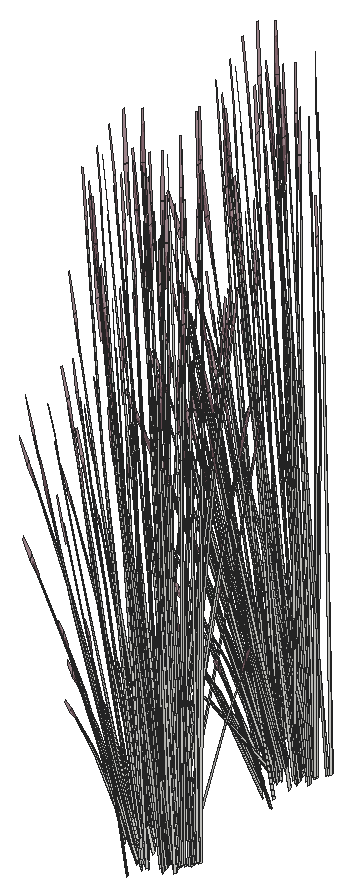
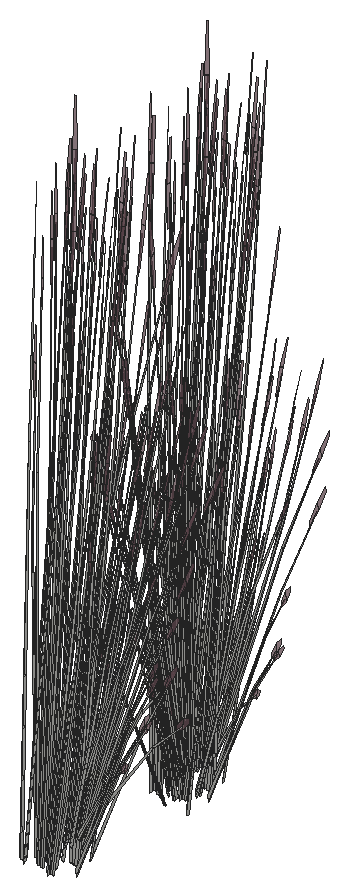
# SketchUp Ruby script. Lengths in inches.
U = 1.inch
M = Sketchup.active_model
def pt(a) = Geom::Point3d.new(a.map { |v| v * U })
def face(e, loops, mat)
  f = e.add_face(loops[0].map { |a| pt(a) })
  loops[1..].each { |l| e.add_face(l.map { |a| pt(a) }).erase! }
  f.material = f.back_material = mat if mat
  f
end
# faces: each face lists its corners as indices into pts; further lists are holes
def faces(e, pts, list, mat = nil) = list.each { |f| face(e, (f[0].is_a?(Array) ? f : [f]).map { |l| l.map { |i| pts[i] } }, mat) }
# xy, xz, yz: faces in a plane at the given z, y or x. An outline is a flat list of corners, or four numbers for a rectangle; further outlines are holes
def ring(l) = l.size == 4 ? [[l[0], l[1]], [l[2], l[1]], [l[2], l[3]], [l[0], l[3]]] : l.each_slice(2).to_a
def flat(e, list, mat, &to3) = list.each { |f| face(e, (f[0].is_a?(Array) ? f : [f]).map { |l| ring(l).map { |u, v| to3.(u, v) } }, mat) }
def xy(e, z, list, mat = nil) = flat(e, list, mat) { |x, y| [x, y, z] }
def xz(e, y, list, mat = nil) = flat(e, list, mat) { |x, z| [x, y, z] }
def yz(e, x, list, mat = nil) = flat(e, list, mat) { |y, z| [x, y, z] }
def lines(e, pts, list) = list.each { |a, b| e.add_line(pt(pts[a]), pt(pts[b])) }
# prism: a flat outline (further loops are holes) pulled along v
def prism(e, loops, v, mat = nil)
  f = face(e, loops, mat); d = Geom::Vector3d.new(v.map { |x| x * U })
  f.pushpull(f.normal.samedirection?(d) ? d.length : -d.length)
end
def box(e, o, s, mat = nil) = prism(e, [[o, [o[0] + s[0], o[1], o[2]], [o[0] + s[0], o[1] + s[1], o[2]], [o[0], o[1] + s[1], o[2]]]], [0, 0, s[2]], mat)
def at(x, y, z, deg = 0) = Geom::Transformation.translation(pt([x, y, z])) * Geom::Transformation.rotation(ORIGIN, Z_AXIS, deg.degrees)
def axes(o, x, y, z) = Geom::Transformation.new([*x, 0, *y, 0, *z, 0, *pt(o).to_a, 1])
def part(name) = M.definitions.add(name)
# library, detail: a bought-in or finely detailed component or shape, given as its bounding box
def library(name, o, s) = part(name).tap { |d| box(d.entities, o, s) }
def detail(e, o, s) = box(e.add_group.entities, o, s)
def put(e, d, t, mat = nil) = e.add_instance(d, t).tap { |i| i.material = mat if mat }
def group(e, t, mat = nil) = e.add_group.tap { |g| g.transformation = t; g.material = mat if mat }.entities
root = M.entities
M.materials.add("LightPink_Translucent").color = [144, 107, 117]
M.materials["LightPink_Translucent"].alpha = 0.75
c1 = part("blade")
p = [[2.15,0.21,22],[0,0.17,0],[0.09,0.45,0],[2.18,0.31,22],[2.29,0.31,22],[0.38,0.45,0],
  [2.48,0.24,33],[2.49,0.24,33],[2.48,0.22,33]]
faces(c1.entities,p,[[0,1,2,3],[4,5,2,3],[6,3,4,7],[8,0,3,6]])
c2 = part("seeds")
p = [[0.3,-0.1,1.38],[-0.01,-0.03,1.59],[-0.01,-0.03,0.03],[0.14,-0.07,-0.07],[0.29,-0.03,3],[0.15,0.01,3.11]]
faces(c2.entities,p,[[0,1,2,3],[1,0,4,5]],"LightPink_Translucent")
c3 = part("blade with seeds")
put(c3.entities,c1,at(0,0,0))
put(c3.entities,c2,axes([2.4,0.25,30.99],[1.5799,-0.05474,1.17369],[-0.12525,1.92788,0.29478],[-0.07173,-0.02425,1.56792]))
put(root,c3,axes([415.25,622.47,157.125],[0.16998,-0.01068,1.44779],[-0.11276,0.46299,0.11706],[-0.24224,-0.02864,0.61892]))
put(root,c3,axes([415.25,635.43,157.55],[0.16998,-0.01068,1.44779],[-0.11276,0.46299,0.11706],[-0.24224,-0.02864,0.61892]))
put(root,c3,axes([415.32,623.29,157.125],[0.14219,-0.09977,1.44779],[0.11971,0.461,0.11706],[-0.22323,0.10419,0.61892]))
put(root,c3,axes([415.32,636.25,157.55],[0.14219,-0.09977,1.44779],[0.11971,0.461,0.11706],[-0.22323,0.10419,0.61892]))
put(root,c3,axes([414.88,624.07,156.04],[0.14242,0.03872,1.20808],[0.09179,0.39548,-0.25981],[-0.19345,0.07403,0.51652]))
put(root,c3,axes([416.14,622.81,156.67],[0.11649,-0.06823,1.49584],[0.04017,0.47639,0.11706],[-0.25231,0.06321,0.53462]))
put(root,c3,axes([416.14,635.77,157.1],[0.11649,-0.06823,1.49584],[0.04017,0.47639,0.11706],[-0.25231,0.06321,0.53462]))
put(root,c3,axes([414.89,623.125,157.83],[-0.06692,0.06124,1.47793],[0.00569,0.44742,-0.23373],[-0.15339,0.05818,0.11853]))
put(root,c3,axes([414.89,636.09,158.26],[-0.06692,0.06124,1.47793],[0.00569,0.44742,-0.23373],[-0.15339,0.05818,0.11853]))
put(root,c3,axes([415.76,622.04,158.06],[-0.40965,-0.01136,-0.60019],[0.02751,-0.47821,0.07243],[-0.17355,-0.05047,0.84903]))
put(root,c3,axes([415.76,635,158.48],[-0.40965,-0.01136,-0.60019],[0.02751,-0.47821,0.07243],[-0.17355,-0.05047,0.84903]))
put(root,c3,axes([415.43,622.16,156.04],[0.08001,0.13132,1.20808],[-0.18437,0.35694,-0.25981],[-0.18931,-0.08532,0.51652]))
put(root,c3,axes([415.43,635.12,156.46],[0.08001,0.13132,1.20808],[-0.18437,0.35694,-0.25981],[-0.18931,-0.08532,0.51652]))
put(root,c3,axes([415.1,622.87,157.68],[-0.34057,-0.13158,-0.29918],[0.09933,-0.38387,0.38624],[-0.13712,0.0352,0.73904]))
put(root,c3,axes([415.1,635.83,158.1],[-0.34057,-0.13158,-0.29918],[0.09933,-0.38387,0.38624],[-0.13712,0.0352,0.73904]))
put(root,c3,axes([415.57,634.69,157.55],[0.15222,0.08126,1.44779],[-0.31502,0.34091,0.11706],[-0.19634,-0.15379,0.61892]))
put(root,c3,axes([414.14,623.58,157.83],[0.0523,0.01265,1.49853],[0.16179,0.41674,-0.1416],[-0.10706,0.10938,0.26519]))
put(root,c3,axes([415.34,623.07,157.81],[-0.11102,0.42903,-0.43168],[-0.38064,-0.14706,-0.33437],[-0.15325,0.03934,0.82598]))
put(root,c3,axes([415.34,636.03,158.23],[-0.11102,0.42903,-0.43168],[-0.38064,-0.14706,-0.33437],[-0.15325,0.03934,0.82598]))
put(root,c3,axes([415.625,622.14,157.81],[-0.29757,0.31243,-0.43168],[-0.2606,-0.33005,-0.33437],[-0.15119,-0.04754,0.82598]))
put(root,c3,axes([415.625,635.1,158.23],[-0.29757,0.31243,-0.43168],[-0.2606,-0.33005,-0.33437],[-0.15119,-0.04754,0.82598]))
put(root,c3,axes([415.14,623.04,155.11],[0.01039,0.07433,1.48974],[-0.20952,0.38819,-0.22758],[-0.14882,-0.01957,0.25375]))
put(root,c3,axes([415.14,636,155.54],[0.01039,0.07433,1.48974],[-0.20952,0.38819,-0.22758],[-0.14882,-0.01957,0.25375]))
put(root,c3,axes([415.2,621.26,157.83],[0.03038,0.04707,1.49853],[-0.14646,0.42312,-0.1416],[-0.14833,0.00306,0.26519]))
put(root,c3,axes([415.2,634.22,158.25],[0.03038,0.04707,1.49853],[-0.14646,0.42312,-0.1416],[-0.14833,0.00306,0.26519]))
put(root,c3,axes([414.58,624.9,156.1875],[0.17079,-0.21377,0.97034],[0.06739,0.33841,0.71294],[-0.12342,0.0606,0.21373]))
put(root,c3,axes([415.54,633.94,158.26],[-0.08817,-0.00333,1.47793],[-0.28072,0.33293,-0.23373],[-0.14978,-0.06803,0.11853]))
put(root,c3,axes([415.18,622.82,157.85],[0.11578,-0.43006,0.40553],[0.38064,0.14706,0.33437],[-0.14969,0.02584,0.83914]))
put(root,c3,axes([415.18,635.78,158.27],[0.11578,-0.43006,0.40553],[0.38064,0.14706,0.33437],[-0.14969,0.02584,0.83914]))
put(root,c3,axes([415.32,622.7,158.1],[0.20619,0.42709,-0.10273],[-0.36595,0.20988,-0.57019],[-0.15422,0.05635,0.8664]))
put(root,c3,axes([415.32,635.66,158.53],[0.20619,0.42709,-0.10273],[-0.36595,0.20988,-0.57019],[-0.15422,0.05635,0.8664]))
put(root,c3,axes([415.78,621.8125,158.1],[-0.02194,0.47967,-0.10273],[-0.41546,-0.01311,-0.57019],[-0.16001,-0.03332,0.8664]))
put(root,c3,axes([415.78,634.77,158.53],[-0.02194,0.47967,-0.10273],[-0.41546,-0.01311,-0.57019],[-0.16001,-0.03332,0.8664]))
put(root,c3,axes([415.51,621.85,157.68],[-0.23317,-0.29531,-0.29918],[0.26625,-0.27955,0.38624],[-0.13527,-0.04253,0.73904]))
put(root,c3,axes([415.51,634.81,158.1],[-0.23317,-0.29531,-0.29918],[0.26625,-0.27955,0.38624],[-0.13527,-0.04253,0.73904]))
put(root,c3,axes([415.15,622.71,157.85],[-0.15051,-0.3216,0.05432],[0.27447,-0.15741,0.42765],[-0.12099,0.03106,0.65209]))
put(root,c3,axes([415.15,635.67,158.27],[-0.15051,-0.3216,0.05432],[0.27447,-0.15741,0.42765],[-0.12099,0.03106,0.65209]))
put(root,c3,axes([415.84,623.6,157.125],[0.10236,-0.14492,1.44779],[0.25844,0.39118,0.11706],[-0.17726,0.17814,0.61892]))
put(root,c3,axes([415.23,623.98,157.68],[-0.35672,0.06741,-0.29918],[-0.09419,-0.38534,0.38624],[-0.10222,0.1035,0.73904]))
put(root,c3,axes([415.03,625.12,155.11],[0.05497,0.04712,1.48974],[0.09321,0.43661,-0.22758],[-0.12183,0.0931,0.25375]))
put(root,c3,axes([414.95,622.55,156.1875],[0.26163,-0.03375,0.97034],[-0.16596,0.29737,0.71294],[-0.12929,-0.04461,0.21373]))
put(root,c3,axes([414.95,635.51,156.61],[0.26163,-0.03375,0.97034],[-0.16596,0.29737,0.71294],[-0.12929,-0.04461,0.21373]))
put(root,c3,axes([415.27,623.9,157.85],[-0.10163,-0.43409,0.40553],[0.39868,-0.07534,0.33437],[-0.1175,0.10209,0.83914]))
put(root,c3,axes([415.27,636.85,158.27],[-0.10163,-0.43409,0.40553],[0.39868,-0.07534,0.33437],[-0.1175,0.10209,0.83914]))
put(root,c3,axes([415.48,634.7,158.58],[0.33843,-0.34808,0.45419],[0.29188,0.36965,0.3745],[-0.15878,-0.06421,0.93983]))
put(root,c3,axes([415.19,623.8125,157.85],[-0.28133,-0.19836,0.05432],[0.16379,-0.28248,0.42765],[-0.0902,0.09132,0.65209]))
put(root,c3,axes([415.19,636.77,158.27],[-0.28133,-0.19836,0.05432],[0.16379,-0.28248,0.42765],[-0.0902,0.09132,0.65209]))
put(root,c3,axes([415.77,623.96,157.125],[0.0763,-0.16212,1.44779],[0.3201,0.3355,0.11706],[-0.1444,0.2091,0.61892]))
put(root,c3,axes([415.46,622.83,158.12],[0.34057,0.13158,0.29918],[-0.09933,0.38387,-0.38624],[-0.13712,0.0352,0.73904]))
put(root,c3,axes([415.46,635.79,158.54],[0.34057,0.13158,0.29918],[-0.09933,0.38387,-0.38624],[-0.13712,0.0352,0.73904]))
put(root,c3,axes([415.52,624.02,157.81],[0.10528,0.43067,-0.43168],[-0.39868,0.07534,-0.33437],[-0.11425,0.11568,0.82598]))
put(root,c3,axes([415.63,621.73,157.85],[0.02064,-0.35866,0.05432],[0.3116,0.00983,0.42765],[-0.11936,-0.03753,0.65209]))
put(root,c3,axes([415.63,634.69,158.27],[0.02064,-0.35866,0.05432],[0.3116,0.00983,0.42765],[-0.11936,-0.03753,0.65209]))
put(root,c3,axes([414.9,624.8,157.83],[-0.01019,0.09334,1.47793],[0.28908,0.3247,-0.23373],[-0.07568,0.15355,0.11853]))
put(root,c3,axes([416.51,623.71,155.59],[-0.42629,-0.07733,-0.52676],[0.08996,-0.47699,-0.13825],[-0.12722,-0.0578,1.16273]))
put(root,c3,axes([416.51,636.67,156.02],[-0.42629,-0.07733,-0.52676],[0.08996,-0.47699,-0.13825],[-0.12722,-0.0578,1.16273]))
put(root,c3,axes([416.59,634.07,158.86],[-0.2735,0.45217,-0.11506],[-0.39608,-0.2605,-0.63862],[-0.13768,-0.12775,0.97037]))
put(root,c3,axes([415.84,622,158.12],[0.23317,0.29531,0.29918],[-0.26625,0.27955,-0.38624],[-0.13527,-0.04253,0.73904]))
put(root,c3,axes([415.84,634.96,158.54],[0.23317,0.29531,0.29918],[-0.26625,0.27955,-0.38624],[-0.13527,-0.04253,0.73904]))
put(root,c3,axes([416.47,634.44,158.48],[-0.34944,-0.22798,-0.60019],[0.24834,-0.39949,0.07243],[-0.1266,-0.13612,0.84903]))
put(root,c3,axes([416.31,634.45,158.23],[-0.40438,0.11212,-0.43168],[-0.07074,-0.4246,-0.33437],[-0.10862,-0.12168,0.82598]))
put(root,c3,axes([415.96,624.62,155.56],[-0.38354,-0.23583,-0.41945],[0.22925,-0.42288,0],[-0.08735,-0.05371,1.33059]))
put(root,c3,axes([415.96,637.58,155.98],[-0.38354,-0.23583,-0.41945],[0.22925,-0.42288,0],[-0.08735,-0.05371,1.33059]))
put(root,c3,axes([415.79,634.06,155.54],[-0.0397,0.06213,1.48974],[-0.40116,0.13396,-0.22758],[-0.09691,-0.12186,0.25375]))
put(root,c3,axes([415.33,623.72,158.1],[0.37908,0.26007,-0.10273],[-0.21839,0.37663,-0.57019],[-0.1071,0.13092,0.8664]))
put(root,c3,axes([416.1875,624.9,155.86],[-0.25622,0.47263,0],[-0.42866,-0.26357,-0.43598],[-0.09763,-0.06003,1.38303]))
put(root,c3,axes([416.1875,637.86,156.28],[-0.25622,0.47263,0],[-0.42866,-0.26357,-0.43598],[-0.09763,-0.06003,1.38303]))
put(root,c3,axes([414.71,624.84,158.62],[0.36162,0.1259,-0.05481],[-0.11124,0.3875,-0.2485],[-0.05915,0.05883,0.81966]))
put(root,c3,axes([415.52,623.75,158.12],[0.35672,-0.06741,0.29918],[0.09419,0.38534,-0.38624],[-0.10222,0.1035,0.73904]))
put(root,c3,axes([415.72,625.59,156.04],[0.12932,-0.07441,1.20808],[0.31929,0.22435,-0.25981],[-0.09503,0.19413,0.51652]))
put(root,c3,axes([415.54,621.34,155.65],[-0.11822,0.38513,-0.03288],[-0.36385,-0.11847,-0.1491],[-0.05524,-0.06299,0.4918]))
put(root,c3,axes([415.54,634.3,156.07],[-0.11822,0.38513,-0.03288],[-0.36385,-0.11847,-0.1491],[-0.05524,-0.06299,0.4918]))
put(root,c3,axes([416.49,633,158.25],[-0.00765,0.05653,1.49853],[-0.37706,0.20517,-0.1416],[-0.11096,-0.10488,0.26519]))
put(root,c3,axes([416.08,633.82,156.46],[-0.02482,0.15429,1.20808],[-0.36278,0.12916,-0.25981],[-0.0848,-0.19943,0.51652]))
put(root,c3,axes([416.2,634.22,157.55],[0.09368,0.15143,1.44779],[-0.43286,0.12749,0.11706],[-0.09783,-0.23774,0.61892]))
put(root,c3,axes([417,623.79,156.1],[-0.41376,0.31314,-0.2458],[-0.27514,-0.44246,-0.42242],[-0.10209,-0.04493,1.34921]))
put(root,c3,axes([417,636.74,156.53],[-0.41376,0.31314,-0.2458],[-0.27514,-0.44246,-0.42242],[-0.10209,-0.04493,1.34921]))
put(root,c3,axes([415.85,624.77,157.85],[-0.29182,-0.32181,0.40553],[0.3099,-0.27755,0.33437],[-0.05383,0.15098,0.83914]))
put(root,c3,axes([416.35,634.14,158.1],[-0.06329,-0.37991,-0.29918],[0.36182,-0.10032,0.38624],[-0.09718,-0.10887,0.73904]))
put(root,c3,axes([415.34,623.1,155.86],[-0.51243,0,0],[0,-0.52715,-0.43598],[0,-0.12006,1.38303]))
put(root,c3,axes([415.34,636.0625,156.28],[-0.51243,0,0],[0,-0.52715,-0.43598],[0,-0.12006,1.38303]))
put(root,c3,axes([416.0625,624.44,155.56],[-0.09626,-0.41098,-0.2617],[0.38233,-0.1167,0.2617],[-0.07708,-0.04739,1.17405]))
put(root,c3,axes([416.0625,637.4,155.99],[-0.09626,-0.41098,-0.2617],[0.38233,-0.1167,0.2617],[-0.07708,-0.04739,1.17405]))
put(root,c3,axes([415.75,624.74,157.85],[-0.33677,-0.02198,0.05432],[0.00923,-0.33185,0.42765],[-0.03524,0.12712,0.65209]))
put(root,c3,axes([415.85,624.87,157.68],[-0.27728,0.24833,-0.29918],[-0.26248,-0.28355,0.38624],[-0.03994,0.14407,0.73904]))
put(root,c3,axes([417.27,624.125,155.59],[-0.27603,0.35451,-0.52676],[-0.34289,-0.32147,-0.13825],[-0.11061,0.08844,1.16273]))
put(root,c3,axes([416.56,634.45,158.54],[0.06329,0.37991,0.29918],[-0.36182,0.10032,-0.38624],[-0.09718,-0.10887,0.73904]))
put(root,c3,axes([414.87,625.75,157.83],[0.04649,-0.02848,1.49853],[0.38427,0.18941,-0.1416],[-0.00903,0.15771,0.26519]))
put(root,c3,axes([415.74,622.96,155.82],[-0.38118,0.39654,0.25983],[-0.38142,-0.39237,-0.30828],[-0.01331,-0.11261,1.39295]))
put(root,c3,axes([415.74,635.92,156.24],[-0.38118,0.39654,0.25983],[-0.38142,-0.39237,-0.30828],[-0.01331,-0.11261,1.39295]))
put(root,c3,axes([417.31,637.02,157.08],[0.35414,0.19019,1.27785],[-0.34693,0.40974,0.50532],[-0.1554,-0.24285,1.07126]))
put(root,c3,axes([415.96,633.57,156.61],[0.21377,0.16416,0.97034],[-0.31132,0.09868,0.71294],[-0.06661,-0.12616,0.21373]))
put(root,c3,axes([417.46,623.93,155.93],[-0.40016,-0.37963,-0.21282],[0.33672,-0.42629,0.46574],[-0.10776,0.04441,1.42109]))
put(root,c3,axes([417.46,636.89,156.36],[-0.40016,-0.37963,-0.21282],[0.33672,-0.42629,0.46574],[-0.10776,0.04441,1.42109]))
put(root,c3,axes([416.74,623.5625,155.72],[-0.24618,-0.39589,-0.37796],[0.37289,-0.27878,0.1819],[-0.07967,-0.04899,1.2135]))
put(root,c3,axes([416.74,636.52,156.14],[-0.24618,-0.39589,-0.37796],[0.37289,-0.27878,0.1819],[-0.07967,-0.04899,1.2135]))
put(root,c3,axes([416.04,624.61,158.36],[-0.01066,0.43628,-0.66621],[-0.44902,-0.0293,0.0804],[-0.04739,0.18483,0.94242]))
put(root,c3,axes([416.03,625.84,156.1875],[-0.01061,-0.28045,0.97034],[0.26501,0.20003,0.71294],[-0.05212,0.13367,0.21373]))
put(root,c3,axes([416.4,634,158.58],[0.45651,-0.12123,0.45419],[0.07923,0.47555,0.3745],[-0.10736,-0.14016,0.93983]))
put(root,c3,axes([417.26,623.85,155.72],[-0.44501,0.02912,-0.37796],[-0.04024,-0.48332,0.1819],[-0.07967,0.04899,1.2135]))
put(root,c3,axes([417.26,636.81,156.14],[-0.44501,0.02912,-0.37796],[-0.04024,-0.48332,0.1819],[-0.07967,0.04899,1.2135]))
put(root,c3,axes([416.51,634.1,158.27],[0.18625,-0.29962,0.05432],[0.26523,0.17444,0.42765],[-0.08575,-0.09606,0.65209]))
put(root,c3,axes([416.41,624.66,155.95],[0.38354,0.23583,0.41945],[-0.22925,0.42288,0],[-0.08735,-0.05371,1.33059]))
put(root,c3,axes([416.41,637.62,156.37],[0.38354,0.23583,0.41945],[-0.22925,0.42288,0],[-0.08735,-0.05371,1.33059]))
put(root,c3,axes([415.89,625.22,156.69],[0.009,-0.24349,1.30391],[0.40497,0.12861,0.18019],[-0.03509,0.2595,0.61571]))
put(root,c3,axes([416.77,623.79,155.91],[0.10862,-0.55889,-0.19793],[0.515,0.09742,0.43313],[-0.08999,-0.07718,1.32161]))
put(root,c3,axes([416.77,636.75,156.34],[0.10862,-0.55889,-0.19793],[0.515,0.09742,0.43313],[-0.08999,-0.07718,1.32161]))
put(root,c3,axes([416.96,623.92,156.0625],[-0.07906,0.42093,0.12232],[-0.38625,-0.07307,-0.3493],[-0.07029,-0.04322,1.07074]))
put(root,c3,axes([416.96,636.88,156.49],[-0.07906,0.42093,0.12232],[-0.38625,-0.07307,-0.3493],[-0.07029,-0.04322,1.07074]))
put(root,c3,axes([416.91,633.21,158.26],[-0.06268,-0.06613,1.47793],[-0.4183,0.04193,-0.23373],[-0.06676,-0.15817,0.11853]))
put(root,c3,axes([417.73,625.09,155.56],[-0.38354,0.23583,-0.41945],[-0.22925,-0.42288,0],[-0.08735,0.05371,1.33059]))
put(root,c3,axes([415.46,635.7,155.98],[0,-0.47166,-0.41945],[0.45849,0,0],[0,-0.10742,1.33059]))
put(root,c3,axes([415.65,623.18,155.95],[0,0.47166,0.41945],[-0.45849,0,0],[0,-0.10742,1.33059]))
put(root,c3,axes([415.65,636.14,156.37],[0,0.47166,0.41945],[-0.45849,0,0],[0,-0.10742,1.33059]))
put(root,c3,axes([417.75,624.97,155.7],[-0.25302,-0.47428,-0.04344],[0.42866,-0.26357,0.43598],[-0.10563,0.04516,1.38235]))
put(root,c3,axes([417.75,637.93,156.13],[-0.25302,-0.47428,-0.04344],[0.42866,-0.26357,0.43598],[-0.10563,0.04516,1.38235]))
put(root,c3,axes([416.13,624.75,158.08],[0.29336,0.31691,-0.47917],[-0.3099,0.27755,-0.37115],[-0.04464,0.16102,0.91684]))
put(root,c3,axes([417.64,624.91,155.56],[-0.38233,-0.1167,-0.2617],[0.09626,-0.41098,0.2617],[-0.07708,0.04739,1.17405]))
put(root,c3,axes([416,624.52,158.12],[0.27728,-0.24833,0.29918],[0.26248,0.28355,-0.38624],[-0.03994,0.14407,0.73904]))
put(root,c3,axes([416.66,623.29,156.1],[-0.46151,-0.22505,-0.2458],[0.22222,-0.475,-0.42242],[-0.0145,-0.11662,1.34921]))
put(root,c3,axes([416.66,636.25,156.53],[-0.46151,-0.22505,-0.2458],[0.22222,-0.475,-0.42242],[-0.0145,-0.11662,1.34921]))
put(root,c3,axes([417.86,623.15,156.25],[-0.01119,-0.44408,1.19347],[0.50665,0.11511,0.50532],[-0.11983,0.243,1.12654]))
put(root,c3,axes([415.82,624.59,158.41],[0.45039,0.02337,-0.11403],[-0.01231,0.44247,-0.63292],[-0.03129,0.17041,0.9617]))
put(root,c3,axes([415.8125,625.23,156.24],[0.37228,-0.08352,0.05498],[0.08559,0.3365,-0.7291],[-0.0236,0.17034,0.65354]))
put(root,c3,axes([417.57,623.72,156.1],[0.04775,0.53819,-0.2458],[-0.49736,0.03254,-0.42242],[-0.08758,0.07169,1.34921]))
put(root,c3,axes([416.45,635.77,156.05],[-0.1683,-0.48366,-0.58997],[0.48479,-0.17419,-0.15484],[-0.0186,-0.16378,1.30225]))
put(root,c3,axes([417.55,634.23,158.53],[-0.40102,0.2196,-0.10273],[-0.19707,-0.38974,-0.57019],[-0.05291,-0.16424,0.8664]))
put(root,c3,axes([417.21,634.25,158.23],[-0.40284,-0.11824,-0.43168],[0.13808,-0.40538,-0.33437],[-0.03694,-0.16321,0.82598]))
put(root,c3,axes([416.46,624.3,157.125],[-0.01003,-0.18103,1.44779],[0.43473,0.12009,0.11706],[-0.02689,0.25798,0.61892]))
put(root,c3,axes([415.65,622.75,155.56],[0.28606,-0.29428,-0.2617],[0.28606,0.29428,0.2617],[0,-0.09479,1.17405]))
put(root,c3,axes([415.65,635.71,155.99],[0.28606,-0.29428,-0.2617],[0.28606,0.29428,0.2617],[0,-0.09479,1.17405]))
put(root,c3,axes([416.95,633.8125,156.07],[-0.28319,0.27058,-0.03288],[-0.25948,-0.29635,-0.1491],[-0.01827,-0.08397,0.4918]))
put(root,c3,axes([416.83,623.52,155.85],[0.51796,0.09937,0.38653],[-0.10541,0.56124,0.15168],[-0.07569,-0.05419,1.34202]))
put(root,c3,axes([416.83,636.48,156.27],[0.51796,0.09937,0.38653],[-0.10541,0.56124,0.15168],[-0.07569,-0.05419,1.34202]))
put(root,c3,axes([416.7,623.42,156.15],[-0.19883,0.425,0.37796],[-0.41314,-0.20454,-0.1819],[0,-0.09797,1.2135]))
put(root,c3,axes([416.7,636.38,156.57],[-0.19883,0.425,0.37796],[-0.41314,-0.20454,-0.1819],[0,-0.09797,1.2135]))
put(root,c3,axes([417.35,634.33,158.48],[-0.19559,-0.38351,-0.60019],[0.40262,-0.21373,0.07243],[-0.04574,-0.1853,0.84903]))
put(root,c3,axes([416.55,624.42,155.94],[0.44036,-0.12519,0.14904],[0.10874,0.46588,0.29641],[-0.03927,-0.06788,1.35512]))
put(root,c3,axes([416.55,637.375,156.37],[0.44036,-0.12519,0.14904],[0.10874,0.46588,0.29641],[-0.03927,-0.06788,1.35512]))
put(root,c3,axes([417.12,624.49,155.71],[-0.41314,-0.21175,0],[0.19883,-0.43999,0],[0,0,1.37455]))
put(root,c3,axes([417.12,637.45,156.13],[-0.41314,-0.21175,0],[0.19883,-0.43999,0],[0,0,1.37455]))
put(root,c3,axes([417.43,634.39,158.54],[-0.12355,0.36271,0.29918],[-0.36044,-0.10579,-0.38624],[-0.03305,-0.14603,0.73904]))
put(root,c3,axes([418.08,625.02,155.86],[0.25622,0.47263,0],[-0.42866,0.26357,-0.43598],[-0.09763,0.06003,1.38303]))
put(root,c3,axes([416.77,625.22,158.13],[-0.4038,-0.12331,0.45013],[0.13808,-0.40538,0.37115],[0.02427,0.15942,0.93144]))
put(root,c3,axes([416.66,625.26,157.85],[-0.30197,0.1603,0.05432],[-0.1478,-0.29231,0.42765],[0.02916,0.12885,0.65209]))
put(root,c3,axes([417.86,624.44,155.94],[0.11838,-0.46875,0.14904],[0.43321,0.13265,0.29641],[-0.07483,0.00228,1.35512]))
put(root,c3,axes([417.86,637.4,156.37],[0.11838,-0.46875,0.14904],[0.43321,0.13265,0.29641],[-0.07483,0.00228,1.35512]))
put(root,c3,axes([417.66,623.82,156.0625],[0.30276,0.28338,0.12232],[-0.25254,0.31972,-0.3493],[-0.07029,0.04322,1.07074]))
put(root,c3,axes([417.66,636.78,156.49],[0.30276,0.28338,0.12232],[-0.25254,0.31972,-0.3493],[-0.07029,0.04322,1.07074]))
put(root,c3,axes([417.56,623.47,155.79],[-0.38118,-0.40596,-0.0518],[0.38142,-0.40621,0],[-0.01331,-0.01418,1.48322]))
put(root,c3,axes([417.56,636.43,156.22],[-0.38118,-0.40596,-0.0518],[0.38142,-0.40621,0],[-0.01331,-0.01418,1.48322]))
put(root,c3,axes([417.66,623.61,156.15],[0.44501,-0.02912,0.37796],[0.04024,0.48332,-0.1819],[-0.07967,0.04899,1.2135]))
put(root,c3,axes([417.66,636.57,156.57],[0.44501,-0.02912,0.37796],[0.04024,0.48332,-0.1819],[-0.07967,0.04899,1.2135]))
put(root,c3,axes([417.76,624.72,155.82],[0.51304,0.1533,0.25983],[-0.12835,0.54797,-0.30828],[-0.08491,0.06858,1.39295]))
put(root,c3,axes([417.02,633.48,155.54],[-0.06874,0.01699,1.48974],[-0.38012,-0.19128,-0.22758],[0.00638,-0.15955,0.25375]))
put(root,c3,axes([417.99,624.69,155.95],[0.38354,-0.23583,0.41945],[0.22925,0.42288,0],[-0.08735,0.05371,1.33059]))
put(root,c3,axes([417.99,637.65,156.37],[0.38354,-0.23583,0.41945],[0.22925,0.42288,0],[-0.08735,0.05371,1.33059]))
put(root,c3,axes([417.39,634.01,158.1],[0.12355,-0.36271,-0.29918],[0.36044,0.10579,0.38624],[-0.03305,-0.14603,0.73904]))
put(root,c3,axes([416.79,623,155.85],[0.17817,0.52741,0.38653],[-0.50909,0.1834,0.15168],[0.00622,-0.09691,1.34202]))
put(root,c3,axes([416.79,635.96,156.27],[0.17817,0.52741,0.38653],[-0.50909,0.1834,0.15168],[0.00622,-0.09691,1.34202]))
put(root,c3,axes([416.7,622.9375,155.72],[0.19883,-0.425,-0.37796],[0.41314,0.20454,0.1819],[0,-0.09797,1.2135]))
put(root,c3,axes([416.7,635.9,156.14],[0.19883,-0.425,-0.37796],[0.41314,0.20454,0.1819],[0,-0.09797,1.2135]))
put(root,c3,axes([417.21,624.31,155.71],[-0.13371,-0.40664,0],[0.38182,-0.1424,0],[0,0,1.30413]))
put(root,c3,axes([417.21,637.27,156.14],[-0.13371,-0.40664,0],[0.38182,-0.1424,0],[0,0,1.30413]))
put(root,c3,axes([416.73,625.17,155.11],[0.06632,-0.02567,1.48974],[0.39894,0.14126,-0.22758],[0.01167,0.15921,0.25375]))
put(root,c3,axes([416.82,625.31,157.68],[-0.12355,0.36271,-0.29918],[-0.36044,-0.10579,0.38624],[0.03305,0.14603,0.73904]))
